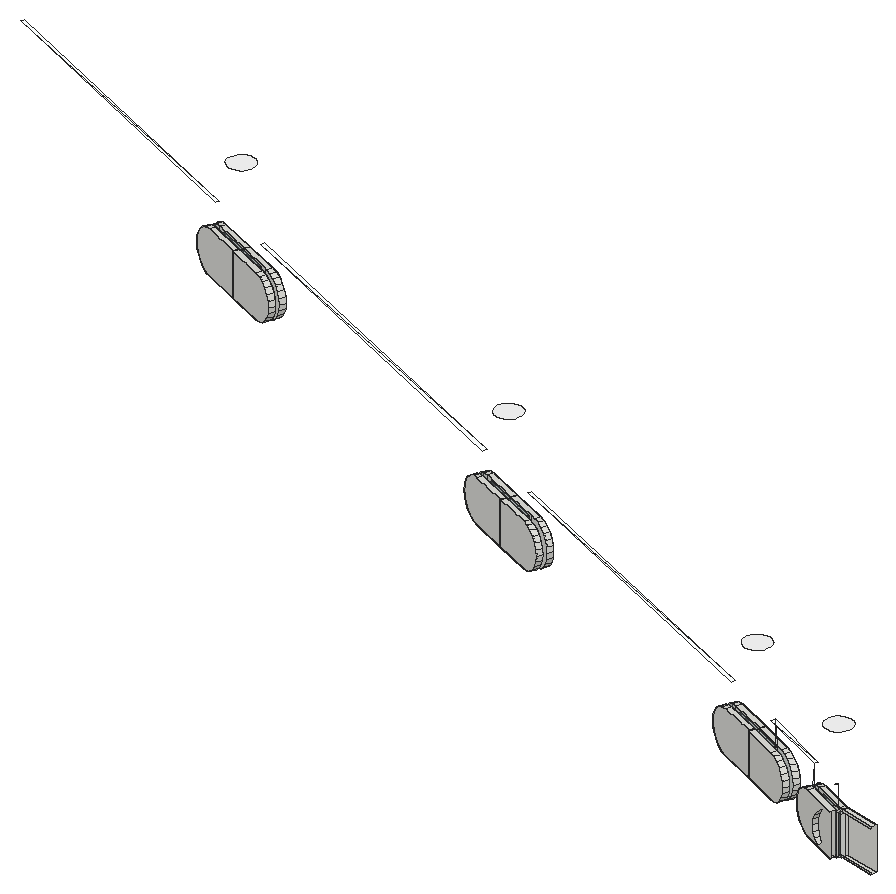
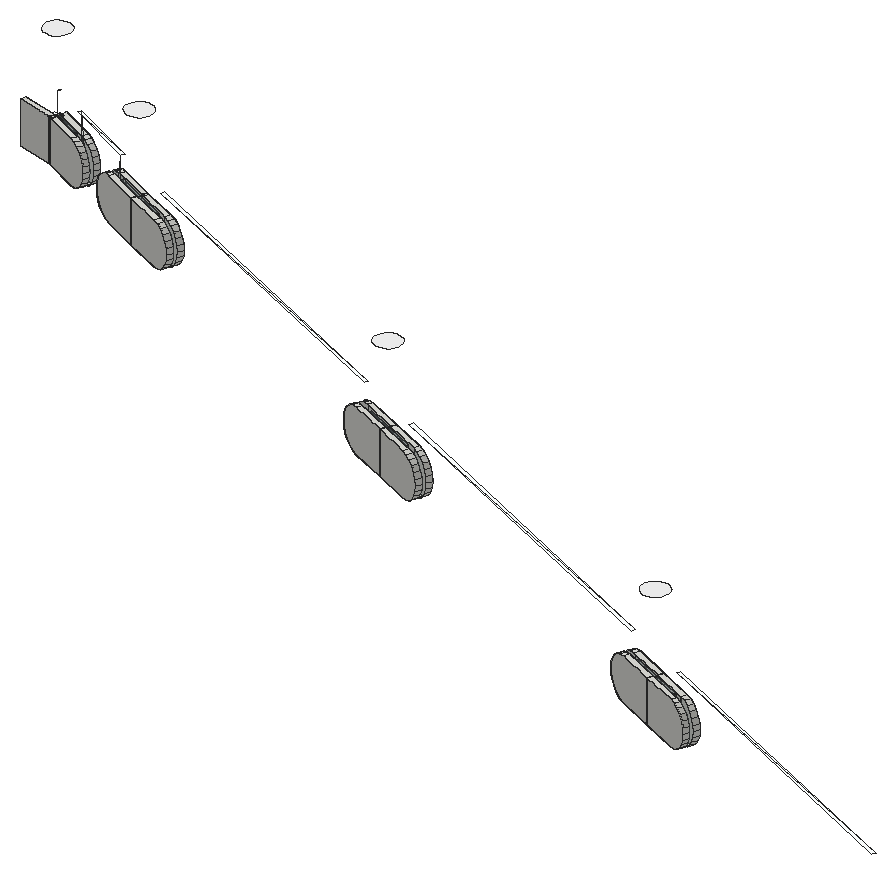
# SketchUp Ruby script. Lengths in inches.
U = 1.inch
M = Sketchup.active_model
def pt(a) = Geom::Point3d.new(a.map { |v| v * U })
def face(e, loops, mat)
  f = e.add_face(loops[0].map { |a| pt(a) })
  loops[1..].each { |l| e.add_face(l.map { |a| pt(a) }).erase! }
  f.material = f.back_material = mat if mat
  f
end
# faces: each face lists its corners as indices into pts; further lists are holes
def faces(e, pts, list, mat = nil) = list.each { |f| face(e, (f[0].is_a?(Array) ? f : [f]).map { |l| l.map { |i| pts[i] } }, mat) }
# xy, xz, yz: faces in a plane at the given z, y or x. An outline is a flat list of corners, or four numbers for a rectangle; further outlines are holes
def ring(l) = l.size == 4 ? [[l[0], l[1]], [l[2], l[1]], [l[2], l[3]], [l[0], l[3]]] : l.each_slice(2).to_a
def flat(e, list, mat, &to3) = list.each { |f| face(e, (f[0].is_a?(Array) ? f : [f]).map { |l| ring(l).map { |u, v| to3.(u, v) } }, mat) }
def xy(e, z, list, mat = nil) = flat(e, list, mat) { |x, y| [x, y, z] }
def xz(e, y, list, mat = nil) = flat(e, list, mat) { |x, z| [x, y, z] }
def yz(e, x, list, mat = nil) = flat(e, list, mat) { |y, z| [x, y, z] }
def lines(e, pts, list) = list.each { |a, b| e.add_line(pt(pts[a]), pt(pts[b])) }
# prism: a flat outline (further loops are holes) pulled along v
def prism(e, loops, v, mat = nil)
  f = face(e, loops, mat); d = Geom::Vector3d.new(v.map { |x| x * U })
  f.pushpull(f.normal.samedirection?(d) ? d.length : -d.length)
end
def box(e, o, s, mat = nil) = prism(e, [[o, [o[0] + s[0], o[1], o[2]], [o[0] + s[0], o[1] + s[1], o[2]], [o[0], o[1] + s[1], o[2]]]], [0, 0, s[2]], mat)
def at(x, y, z, deg = 0) = Geom::Transformation.translation(pt([x, y, z])) * Geom::Transformation.rotation(ORIGIN, Z_AXIS, deg.degrees)
def axes(o, x, y, z) = Geom::Transformation.new([*x, 0, *y, 0, *z, 0, *pt(o).to_a, 1])
def part(name) = M.definitions.add(name)
# library, detail: a bought-in or finely detailed component or shape, given as its bounding box
def library(name, o, s) = part(name).tap { |d| box(d.entities, o, s) }
def detail(e, o, s) = box(e.add_group.entities, o, s)
def put(e, d, t, mat = nil) = e.add_instance(d, t).tap { |i| i.material = mat if mat }
def group(e, t, mat = nil) = e.add_group.tap { |g| g.transformation = t; g.material = mat if mat }.entities
root = M.entities
M.materials.add("Glass_Safety_01").color = [204, 235, 244]
M.materials["Glass_Safety_01"].alpha = 0.1
M.materials.add("[Color_000]").color = [255, 255, 255]
xy(root,351.283,[[1021.879,1012.714,1020.123,1013.542,1020.24,1013.791,1022.021,1012.952,1022.02,1012.949,1021.935,1012.968],[1023.9,1012.74,1022.106,1013.132,1022.222,1013.379,1022.184,1013.397,1023.959,1013.009],[1022.105,1013.13,1022.095,1013.134,1022.106,1013.132],[1022.106,1013.132,1022.095,1013.134,1021.983,1013.1875,1022.035,1013.429,1022.184,1013.397,1022.222,1013.379],[1022.095,1013.134,1022.084,1013.137,1021.977,1013.16,1021.983,1013.1875],
  [1021.983,1013.1875,1020.324,1013.969,1020.442,1014.219,1022.184,1013.397,1022.035,1013.429],[1017.116,1014.96,1015.346,1015.795,1015.456,1016.048,1016.751,1015.437,1017.234,1015.209],[1017.318,1015.387,1016.835,1015.615,1015.537,1016.227,1015.655,1016.476,1017.435,1015.637],[1015.346,1015.795,1015.341,1015.797,1015.336,1015.8,1015.453,1016.049,1015.456,1016.048],[1015.336,1015.8,1013.541,1016.581,1013.651,1016.834,1015.453,1016.049],
  [1015.535,1016.228,1013.73,1017.014,1013.84,1017.267,1015.645,1016.481],[998.018,1023.342,996.213,1024.128,996.324,1024.38,997.958,1023.669,998.128,1023.594],[998.207,1023.775,998.037,1023.849,996.402,1024.561,996.512,1024.814,998.317,1024.028],[996.213,1024.128,994.409,1024.914,994.519,1025.167,996.324,1024.38],[996.402,1024.561,994.597,1025.347,994.707,1025.6,996.512,1024.814],
  [977.436,1032.306,975.631,1033.092,975.741,1033.345,977.388,1032.628,977.546,1032.559],[977.625,1032.739,977.466,1032.808,975.82,1033.525,975.93,1033.778,977.735,1032.992],[975.631,1033.092,973.826,1033.878,973.936,1034.131,975.741,1033.345],[975.82,1033.525,974.015,1034.311,974.125,1034.564,975.93,1033.778]])
xy(root,351.362,[[1022.319,1012.884,1022.042,1012.945,1022.063,1013.041,1022.105,1013.13,1022.095,1013.134,1022.361,1013.076],[1022.021,1012.952,1020.597,1013.623,1020.681,1013.801,1022.095,1013.134,1022.084,1013.137,1022.063,1013.041],[1022.063,1013.041,1022.084,1013.137,1022.095,1013.134,1022.105,1013.13],[1016.878,1015.377,1016.751,1015.437,1015.456,1016.048,1015.495,1016.138,1015.537,1016.227,1016.835,1015.615,1016.962,1015.555],[1015.455,1016.048,1015.453,1016.049,1015.495,1016.138,1015.456,1016.048],
  [1015.453,1016.049,1014.012,1016.677,1014.091,1016.857,1015.535,1016.228,1015.495,1016.138],[997.767,1023.752,996.324,1024.38,996.402,1024.561,997.846,1023.932],[996.324,1024.38,994.88,1025.009,994.958,1025.19,996.402,1024.561],[977.185,1032.716,975.741,1033.345,975.82,1033.525,977.264,1032.896],[975.741,1033.345,974.297,1033.974,974.376,1034.154,975.82,1033.525]],"Glass_Safety_01")
xy(root,353.33,[[1022.319,1012.884,1022.361,1013.076,1022.095,1013.134,1022.105,1013.13,1022.063,1013.041,1022.042,1012.945],[1022.021,1012.952,1022.063,1013.041,1022.084,1013.137,1022.095,1013.134,1020.681,1013.801,1020.597,1013.623],[1022.063,1013.041,1022.105,1013.13,1022.095,1013.134,1022.084,1013.137],[1016.878,1015.377,1016.962,1015.555,1016.835,1015.615,1015.537,1016.227,1015.495,1016.138,1015.456,1016.048,1016.751,1015.437],[1015.455,1016.048,1015.456,1016.048,1015.495,1016.138,1015.453,1016.049],
  [1015.453,1016.049,1015.495,1016.138,1015.535,1016.228,1014.091,1016.857,1014.012,1016.677],[997.767,1023.752,997.846,1023.932,996.402,1024.561,996.324,1024.38],[996.324,1024.38,996.402,1024.561,994.958,1025.19,994.88,1025.009],[977.185,1032.716,977.264,1032.896,975.82,1033.525,975.741,1033.345],[975.741,1033.345,975.82,1033.525,974.376,1034.154,974.297,1033.974]],"Glass_Safety_01")
xy(root,353.409,[[1021.879,1012.714,1021.935,1012.968,1022.02,1012.949,1022.021,1012.952,1020.24,1013.791,1020.123,1013.542],[1023.9,1012.74,1023.959,1013.009,1022.184,1013.397,1022.222,1013.379,1022.106,1013.132],[1022.105,1013.13,1022.106,1013.132,1022.095,1013.134],[1022.106,1013.132,1022.222,1013.379,1022.184,1013.397,1022.035,1013.429,1021.983,1013.1875,1022.095,1013.134],[1022.095,1013.134,1021.983,1013.1875,1021.977,1013.16,1022.084,1013.137],
  [1021.983,1013.1875,1022.035,1013.429,1022.184,1013.397,1020.442,1014.219,1020.324,1013.969],[1017.116,1014.96,1017.234,1015.209,1016.751,1015.437,1015.456,1016.048,1015.346,1015.795],[1017.318,1015.387,1017.435,1015.637,1015.655,1016.476,1015.537,1016.227,1016.835,1015.615,1017.005,1015.535],[1015.346,1015.795,1015.456,1016.048,1015.453,1016.049,1015.336,1015.8,1015.341,1015.797],[1015.336,1015.8,1015.453,1016.049,1013.651,1016.834,1013.541,1016.581],
  [1015.535,1016.228,1015.645,1016.481,1013.84,1017.267,1013.73,1017.014],[998.018,1023.342,998.128,1023.594,997.958,1023.669,996.324,1024.38,996.213,1024.128],[998.207,1023.775,998.317,1024.028,996.512,1024.814,996.402,1024.561,998.037,1023.849],[996.213,1024.128,996.324,1024.38,994.519,1025.167,994.409,1024.914],[996.402,1024.561,996.512,1024.814,994.707,1025.6,994.597,1025.347],
  [977.436,1032.306,977.546,1032.559,977.388,1032.628,975.741,1033.345,975.631,1033.092],[977.625,1032.739,977.735,1032.992,975.93,1033.778,975.82,1033.525,977.466,1032.808],[975.631,1033.092,975.741,1033.345,973.936,1034.131,973.826,1033.878],[975.82,1033.525,975.93,1033.778,974.125,1034.564,974.015,1034.311]])
xy(root,354.511,[[1021.935,1012.968,1021.977,1013.16,1021.928,1012.969],[1021.928,1012.969,1021.977,1013.16,1021.97,1013.162],[1020.24,1013.791,1020.324,1013.969,1016.751,1015.437],[1020.324,1013.969,1016.835,1015.615,1016.751,1015.437],[1013.651,1016.834,1013.73,1017.014,997.958,1023.669],
  [1013.73,1017.014,998.037,1023.849,997.958,1023.669],[994.519,1025.167,994.597,1025.347,977.388,1032.628],[994.597,1025.347,977.466,1032.808,977.388,1032.628],[973.936,1034.131,974.015,1034.311,958.914,1040.674],[974.015,1034.311,958.992,1040.854,958.914,1040.674]],"Glass_Safety_01")
xy(root,357.267,[[1022.108,1012.412,1022.269,1012.445,1022.416,1012.519,1022.539,1012.628,1022.63,1012.766,1022.681,1012.922,1022.691,1013.086,1022.658,1013.247,1022.584,1013.394,1022.475,1013.517,1022.338,1013.607,1022.182,1013.659,1022.018,1013.669,1021.857,1013.636,1021.71,1013.562,1021.587,1013.453,1021.496,1013.316,1021.444,1013.16,1021.435,1012.996,1021.468,1012.835,1021.541,1012.6875,1021.65,1012.565,1021.788,1012.474,1021.944,1012.422],[1015.54,1015.51,1015.701,1015.543,1015.848,1015.616,1015.971,1015.726,1016.062,1015.863,1016.114,1016.019,1016.124,1016.183,1016.09,1016.344,1016.017,1016.491,1015.908,1016.614,1015.77,1016.705,1015.614,1016.757,1015.45,1016.766,1015.289,1016.733,1015.142,1016.66,1015.019,1016.55,1014.929,1016.413,1014.877,1016.257,1014.867,1016.093,1014.9,1015.932,1014.974,1015.785,1015.083,1015.662,1015.22,1015.571,1015.376,1015.519],[996.408,1023.842,996.569,1023.875,996.716,1023.949,996.839,1024.058,996.929,1024.196,996.981,1024.352,996.991,1024.516,996.958,1024.677,996.884,1024.824,996.775,1024.947,996.638,1025.037,996.482,1025.089,996.318,1025.099,996.157,1025.066,996.01,1024.992,995.887,1024.883,995.796,1024.746,995.744,1024.59,995.735,1024.426,995.768,1024.265,995.841,1024.118,995.95,1023.995,996.088,1023.904,996.244,1023.852],[975.826,1032.807,975.987,1032.84,976.134,1032.913,976.257,1033.023,976.347,1033.16,976.399,1033.316,976.409,1033.48,976.376,1033.641,976.302,1033.788,976.193,1033.911,976.056,1034.002,975.9,1034.054,975.735,1034.063,975.574,1034.03,975.427,1033.957,975.304,1033.847,975.214,1033.71,975.162,1033.554,975.152,1033.39,975.185,1033.229,975.259,1033.082,975.368,1032.959,975.505,1032.868,975.661,1032.816]],"[Color_000]")
p = [[1021.903,1012.702,353.409],[1021.879,1012.714,353.409],[1020.123,1013.542,353.409],[1019.874,1013.659,353.373],[1019.642,1013.769,353.267],[1019.443,1013.863,353.098],
  [1019.29,1013.935,352.877],[1019.194,1013.98,352.621],[1019.161,1013.995,352.346],[1019.194,1013.98,352.071],[1019.29,1013.935,351.814],[1019.443,1013.863,351.594],
  [1019.642,1013.769,351.425],[1019.874,1013.659,351.319],[1020.123,1013.542,351.283],[1021.879,1012.714,351.283],[1021.903,1012.702,351.283],[1022.095,1013.134,351.362],
  [1022.361,1013.076,351.362],[1023.622,1012.801,351.362],[1023.9,1012.74,351.362],[1023.9,1012.74,351.283],[1022.106,1013.132,351.283],[1022.095,1013.134,351.283],
  [1022.084,1013.137,351.283],[1022.084,1013.137,351.362],[1022.063,1013.041,351.362],[1022.042,1012.945,351.362],[1022.042,1012.945,351.283],[1022.021,1012.952,351.283],
  [1020.24,1013.791,351.283],[1020.24,1013.791,353.409],[1022.021,1012.952,353.409],[1022.021,1012.952,353.33],[1020.597,1013.623,353.33],[1020.597,1013.623,351.362],
  [1022.021,1012.952,351.362],[1021.666,1013.027,353.373],[1021.928,1012.969,353.408],[1021.928,1012.969,351.284],[1021.666,1013.027,351.319],[1021.415,1013.081,351.425],
  [1021.2,1013.128,351.594],[1021.035,1013.164,351.814],[1020.932,1013.187,352.071],[1020.896,1013.195,352.346],[1020.932,1013.187,352.621],[1021.035,1013.164,352.877],
  [1021.2,1013.128,353.098],[1021.415,1013.081,353.267],[1022.184,1013.397,353.409],[1023.959,1013.009,353.409],[1023.959,1013.009,351.283],[1022.184,1013.397,351.283],
  [1022.035,1013.429,351.283],[1021.767,1013.488,351.319],[1021.516,1013.543,351.425],[1021.301,1013.59,351.594],[1021.136,1013.626,351.814],[1021.032,1013.649,352.071],
  [1020.997,1013.656,352.346],[1021.032,1013.649,352.621],[1021.136,1013.626,352.877],[1021.301,1013.59,353.098],[1021.516,1013.543,353.267],[1021.767,1013.488,353.373],
  [1022.035,1013.429,353.409],[1021.983,1013.1875,353.409],[1020.324,1013.969,353.409],[1020.324,1013.969,351.283],[1021.983,1013.1875,351.283],[1022.105,1013.13,351.283],
  [1022.105,1013.13,351.362],[1020.681,1013.801,351.362],[1020.681,1013.801,353.33],[1022.095,1013.134,353.33],[1022.105,1013.13,353.33],[1022.105,1013.13,353.409],
  [1022.095,1013.134,353.409],[1022.084,1013.137,353.409],[1021.977,1013.16,353.409],[1021.977,1013.16,351.283],[1022.084,1013.137,353.33],[1022.222,1013.379,351.283],
  [1022.222,1013.379,353.409],[1022.106,1013.132,353.409],[1021.708,1013.219,351.319],[1021.971,1013.161,351.284],[1021.971,1013.162,353.408],[1021.708,1013.219,353.373],
  [1021.457,1013.274,353.267],[1021.242,1013.321,353.098],[1021.077,1013.357,352.877],[1020.974,1013.379,352.621],[1020.938,1013.387,352.346],[1020.974,1013.379,352.071],
  [1021.077,1013.357,351.814],[1021.242,1013.321,351.594],[1021.457,1013.274,351.425],[1020.442,1014.219,351.283],[1020.193,1014.336,351.319],[1019.961,1014.445,351.425],
  [1019.762,1014.539,351.594],[1019.609,1014.611,351.814],[1019.513,1014.657,352.071],[1019.481,1014.672,352.346],[1019.513,1014.657,352.621],[1019.609,1014.611,352.877],
  [1019.762,1014.539,353.098],[1019.961,1014.445,353.267],[1020.193,1014.336,353.373],[1020.442,1014.219,353.409],[1019.992,1013.909,351.319],[1019.76,1014.018,351.425],
  [1019.764,1014.016,351.423],[1020.066,1013.873,353.384],[1020.076,1014.087,351.319],[1019.844,1014.196,351.425],[1019.645,1014.29,351.594],[1019.492,1014.362,351.814],
  [1019.396,1014.407,352.071],[1019.363,1014.423,352.346],[1019.396,1014.407,352.621],[1019.492,1014.362,352.877],[1019.645,1014.29,353.098],[1019.844,1014.196,353.267],
  [1020.076,1014.087,353.373],[1017.116,1014.96,353.409],[1015.346,1015.795,353.409],[1015.346,1015.795,351.283],[1017.116,1014.96,351.283],[1017.365,1014.843,351.319],
  [1017.597,1014.733,351.425],[1017.796,1014.639,351.594],[1017.949,1014.567,351.814],[1018.045,1014.522,352.071],[1018.078,1014.507,352.346],[1018.045,1014.522,352.621],
  [1017.949,1014.567,352.877],[1017.796,1014.639,353.098],[1017.597,1014.733,353.267],[1017.365,1014.843,353.373],[1017.483,1015.092,351.319],[1017.714,1014.983,351.425],
  [1016.751,1015.437,351.362],[1016.751,1015.437,351.283],[1017.234,1015.209,351.283],[1017.914,1014.889,351.594],[1018.066,1014.817,351.814],[1018.162,1014.771,352.071],
  [1018.195,1014.756,352.346],[1018.162,1014.771,352.621],[1018.066,1014.817,352.877],[1017.914,1014.889,353.098],[1017.714,1014.983,353.267],[1017.483,1015.092,353.373],
  [1017.234,1015.209,353.409],[1016.751,1015.437,353.409],[1016.751,1015.437,353.33],[1016.878,1015.377,353.33],[1016.878,1015.377,351.362],[1017.005,1015.535,353.409],
  [1017.333,1015.38,351.285],[1017.567,1015.27,351.319],[1017.798,1015.161,351.425],[1017.998,1015.067,351.594],[1018.15,1014.995,351.814],[1018.246,1014.949,352.071],
  [1018.279,1014.934,352.346],[1018.246,1014.949,352.621],[1018.15,1014.995,352.877],[1017.998,1015.067,353.098],[1017.798,1015.161,353.267],[1017.567,1015.27,353.373],
  [1017.318,1015.387,353.409],[1015.655,1016.476,353.409],[1017.435,1015.637,353.409],[1017.684,1015.519,353.373],[1017.916,1015.41,353.267],[1018.115,1015.316,353.098],
  [1018.268,1015.244,352.877],[1018.364,1015.199,352.621],[1018.397,1015.183,352.346],[1018.364,1015.199,352.071],[1018.268,1015.244,351.814],[1018.115,1015.316,351.594],
  [1017.916,1015.41,351.425],[1017.684,1015.519,351.319],[1017.435,1015.637,351.283],[1015.655,1016.476,351.283],[1017.318,1015.387,351.283],[1015.456,1016.048,351.283],
  [1015.456,1016.048,351.362],[1016.835,1015.615,353.409],[1016.835,1015.615,353.33],[1016.962,1015.555,353.33],[1016.962,1015.555,351.362],[1016.835,1015.615,351.362],
  [1016.835,1015.615,351.283],[1015.537,1016.227,351.283],[1015.537,1016.227,351.362],[1015.341,1015.797,353.409],[1015.336,1015.8,353.409],[1013.541,1016.581,353.409],
  [1013.289,1016.691,353.373],[1013.054,1016.793,353.267],[1012.852,1016.881,353.098],[1012.697,1016.949,352.877],[1012.6,1016.991,352.621],[1012.567,1017.006,352.346],
  [1012.6,1016.991,352.071],[1012.697,1016.949,351.814],[1012.852,1016.881,351.594],[1013.054,1016.793,351.425],[1013.289,1016.691,351.319],[1013.541,1016.581,351.283],
  [1015.336,1015.8,351.283],[1015.341,1015.797,351.283],[1015.456,1016.048,353.33],[1015.456,1016.048,353.409],[1015.453,1016.049,351.362],[1015.453,1016.049,351.283],
  [1015.453,1016.049,353.409],[1015.453,1016.049,353.33],[1013.651,1016.834,353.409],[1014.012,1016.677,353.33],[1014.012,1016.677,351.362],[1013.651,1016.834,351.283],
  [1013.399,1016.944,351.319],[1013.164,1017.046,351.425],[1012.962,1017.134,351.594],[1012.807,1017.201,351.814],[1012.71,1017.244,352.071],[1012.677,1017.258,352.346],
  [1012.71,1017.244,352.621],[1012.807,1017.201,352.877],[1012.962,1017.134,353.098],[1013.164,1017.046,353.267],[1013.399,1016.944,353.373],[1015.455,1016.048,351.362],
  [1015.535,1016.228,353.409],[1013.73,1017.014,353.409],[1013.73,1017.014,351.283],[1015.535,1016.228,351.283],[1015.535,1016.228,351.362],[1014.091,1016.857,351.362],
  [1014.091,1016.857,353.33],[1015.535,1016.228,353.33],[1015.537,1016.227,353.33],[1015.537,1016.227,353.409],[1015.645,1016.481,351.283],[1015.645,1016.481,353.409],
  [1013.84,1017.267,353.409],[1013.84,1017.267,351.283],[1013.588,1017.377,351.319],[1013.353,1017.479,351.425],[1013.151,1017.567,351.594],[1012.996,1017.635,351.814],
  [1012.898,1017.677,352.071],[1012.865,1017.691,352.346],[1012.898,1017.677,352.621],[1012.996,1017.635,352.877],[1013.151,1017.567,353.098],[1013.353,1017.479,353.267],
  [1013.588,1017.377,353.373],[1013.478,1017.124,351.319],[1013.242,1017.226,351.425],[1013.041,1017.314,351.594],[1012.886,1017.382,351.814],[1012.788,1017.424,352.071],
  [1012.755,1017.439,352.346],[1012.788,1017.424,352.621],[1012.886,1017.382,352.877],[1013.041,1017.314,353.098],[1013.242,1017.226,353.267],[1013.478,1017.124,353.373],
  [998.018,1023.342,353.409],[996.213,1024.128,353.409],[996.213,1024.128,351.283],[998.018,1023.342,351.283],[998.27,1023.232,351.319],[998.506,1023.13,351.425],
  [998.707,1023.042,351.594],[998.862,1022.974,351.814],[998.96,1022.932,352.071],[998.993,1022.917,352.346],[998.96,1022.932,352.621],[998.862,1022.974,352.877],
  [998.707,1023.042,353.098],[998.506,1023.13,353.267],[998.27,1023.232,353.373],[998.381,1023.485,351.319],[998.616,1023.382,351.425],[998.128,1023.594,351.283],
  [997.958,1023.669,351.283],[997.958,1023.669,353.409],[998.128,1023.594,353.409],[998.381,1023.485,353.373],[998.616,1023.382,353.267],[998.817,1023.294,353.098],
  [998.972,1023.227,352.877],[999.07,1023.184,352.621],[999.103,1023.17,352.346],[999.07,1023.184,352.071],[998.972,1023.227,351.814],[998.817,1023.294,351.594],
  [998.207,1023.775,353.409],[998.037,1023.849,353.409],[998.037,1023.849,351.283],[998.207,1023.775,351.283],[998.459,1023.665,351.319],[998.694,1023.563,351.425],
  [998.896,1023.475,351.594],[999.051,1023.407,351.814],[999.148,1023.365,352.071],[999.181,1023.35,352.346],[999.148,1023.365,352.621],[999.051,1023.407,352.877],
  [998.896,1023.475,353.098],[998.694,1023.563,353.267],[998.459,1023.665,353.373],[996.512,1024.814,353.409],[998.317,1024.028,353.409],[998.569,1023.918,353.373],
  [998.804,1023.815,353.267],[999.006,1023.727,353.098],[999.161,1023.66,352.877],[999.258,1023.618,352.621],[999.291,1023.603,352.346],[999.258,1023.618,352.071],
  [999.161,1023.66,351.814],[999.006,1023.727,351.594],[998.804,1023.815,351.425],[998.569,1023.918,351.319],[998.317,1024.028,351.283],[996.512,1024.814,351.283],
  [996.324,1024.38,353.409],[996.324,1024.38,351.283],[996.324,1024.38,351.362],[997.767,1023.752,351.362],[997.767,1023.752,353.33],[996.324,1024.38,353.33],
  [996.402,1024.561,351.283],[996.402,1024.561,353.409],[996.402,1024.561,353.33],[997.846,1023.932,353.33],[997.846,1023.932,351.362],[996.402,1024.561,351.362],
  [994.409,1024.914,353.409],[994.156,1025.024,353.373],[993.921,1025.126,353.267],[993.72,1025.214,353.098],[993.565,1025.281,352.877],[993.467,1025.324,352.621],
  [993.434,1025.338,352.346],[993.467,1025.324,352.071],[993.565,1025.281,351.814],[993.72,1025.214,351.594],[993.921,1025.126,351.425],[994.156,1025.024,351.319],
  [994.409,1024.914,351.283],[994.519,1025.167,351.283],[994.519,1025.167,353.409],[994.88,1025.009,353.33],[994.88,1025.009,351.362],[994.597,1025.347,353.409],
  [994.597,1025.347,351.283],[994.958,1025.19,351.362],[994.958,1025.19,353.33],[994.707,1025.6,353.409],[994.707,1025.6,351.283],[994.455,1025.71,351.319],
  [994.22,1025.812,351.425],[994.018,1025.9,351.594],[993.863,1025.967,351.814],[993.766,1026.01,352.071],[993.733,1026.024,352.346],[993.766,1026.01,352.621],
  [993.863,1025.967,352.877],[994.018,1025.9,353.098],[994.22,1025.812,353.267],[994.455,1025.71,353.373],[994.267,1025.276,351.319],[994.031,1025.379,351.425],
  [994.267,1025.276,353.373],[994.031,1025.379,353.267],[993.83,1025.467,353.098],[993.675,1025.534,352.877],[993.577,1025.577,352.621],[993.544,1025.591,352.346],
  [993.577,1025.577,352.071],[993.675,1025.534,351.814],[993.83,1025.467,351.594],[994.345,1025.457,351.319],[994.11,1025.559,351.425],[993.908,1025.647,351.594],
  [993.753,1025.715,351.814],[993.656,1025.757,352.071],[993.623,1025.771,352.346],[993.656,1025.757,352.621],[993.753,1025.715,352.877],[993.908,1025.647,353.098],
  [994.11,1025.559,353.267],[994.345,1025.457,353.373],[977.436,1032.306,353.409],[975.631,1033.092,353.409],[975.631,1033.092,351.283],[977.436,1032.306,351.283],
  [977.688,1032.196,351.319],[977.923,1032.094,351.425],[978.125,1032.006,351.594],[978.28,1031.938,351.814],[978.377,1031.896,352.071],[978.41,1031.882,352.346],
  [978.377,1031.896,352.621],[978.28,1031.938,352.877],[978.125,1032.006,353.098],[977.923,1032.094,353.267],[977.688,1032.196,353.373],[977.546,1032.559,351.283],
  [977.388,1032.628,351.283],[977.388,1032.628,353.409],[977.546,1032.559,353.409],[977.798,1032.449,353.373],[978.033,1032.346,353.267],[978.235,1032.259,353.098],
  [978.39,1032.191,352.877],[978.487,1032.149,352.621],[978.521,1032.134,352.346],[978.487,1032.149,352.071],[978.39,1032.191,351.814],[978.235,1032.259,351.594],
  [978.033,1032.346,351.425],[977.798,1032.449,351.319],[977.625,1032.739,353.409],[977.466,1032.808,353.409],[977.466,1032.808,351.283],[977.625,1032.739,351.283],
  [977.877,1032.629,351.319],[978.112,1032.527,351.425],[978.314,1032.439,351.594],[978.469,1032.372,351.814],[978.566,1032.329,352.071],[978.599,1032.315,352.346],
  [978.566,1032.329,352.621],[978.469,1032.372,352.877],[978.314,1032.439,353.098],[978.112,1032.527,353.267],[977.877,1032.629,353.373],[977.987,1032.882,351.319],
  [978.222,1032.78,351.425],[975.741,1033.345,353.409],[975.741,1033.345,351.283],[975.741,1033.345,351.362],[977.185,1032.716,351.362],[977.185,1032.716,353.33],
  [975.741,1033.345,353.33],[975.93,1033.778,353.409],[977.735,1032.992,353.409],[977.987,1032.882,353.373],[978.222,1032.78,353.267],[978.424,1032.692,353.098],
  [978.579,1032.624,352.877],[978.676,1032.582,352.621],[978.709,1032.567,352.346],[978.676,1032.582,352.071],[978.579,1032.624,351.814],[978.424,1032.692,351.594],
  [977.735,1032.992,351.283],[975.93,1033.778,351.283],[975.82,1033.525,351.283],[975.82,1033.525,353.409],[975.82,1033.525,353.33],[977.264,1032.896,353.33],
  [977.264,1032.896,351.362],[975.82,1033.525,351.362],[973.826,1033.878,353.409],[973.574,1033.988,353.373],[973.339,1034.09,353.267],[973.137,1034.178,353.098],
  [972.982,1034.246,352.877],[972.885,1034.288,352.621],[972.852,1034.303,352.346],[972.885,1034.288,352.071],[972.982,1034.246,351.814],[973.137,1034.178,351.594],
  [973.339,1034.09,351.425],[973.574,1033.988,351.319],[973.826,1033.878,351.283],[973.936,1034.131,351.283],[973.936,1034.131,353.409],[974.297,1033.974,353.33],
  [974.297,1033.974,351.362],[974.015,1034.311,353.409],[974.015,1034.311,351.283],[974.376,1034.154,351.362],[974.376,1034.154,353.33],[974.125,1034.564,353.409],
  [974.125,1034.564,351.283],[973.873,1034.674,351.319],[973.638,1034.776,351.425],[973.436,1034.864,351.594],[973.281,1034.931,351.814],[973.184,1034.974,352.071],
  [973.15,1034.988,352.346],[973.184,1034.974,352.621],[973.281,1034.931,352.877],[973.436,1034.864,353.098],[973.638,1034.776,353.267],[973.873,1034.674,353.373],
  [973.684,1034.241,351.319],[973.449,1034.343,351.425],[973.684,1034.241,353.373],[973.449,1034.343,353.267],[973.247,1034.431,353.098],[973.092,1034.498,352.877],
  [972.995,1034.541,352.621],[972.962,1034.555,352.346],[972.995,1034.541,352.071],[973.092,1034.498,351.814],[973.247,1034.431,351.594],[973.763,1034.421,351.319],
  [973.528,1034.523,351.425],[973.326,1034.611,351.594],[973.171,1034.679,351.814],[973.074,1034.721,352.071],[973.04,1034.736,352.346],[973.074,1034.721,352.621],
  [973.171,1034.679,352.877],[973.326,1034.611,353.098],[973.528,1034.523,353.267],[973.763,1034.421,353.373],[1022.063,1013.041,353.33],[1022.042,1012.945,353.33],
  [1022.361,1013.076,353.33],[1019.561,1014.112,351.594],[1019.992,1013.909,353.373],[1019.76,1014.018,353.267],[1019.561,1014.112,353.098],[1019.408,1014.184,352.877],
  [1019.312,1014.229,352.621],[1019.279,1014.245,352.346],[1019.312,1014.229,352.071],[1019.408,1014.184,351.814],[1015.455,1016.048,353.33],[1015.495,1016.138,351.362],
  [1015.495,1016.138,353.33],[1021.141,1012.859,351.594],[1020.976,1012.895,351.814],[1020.873,1012.918,352.071],[1020.837,1012.926,352.346],[1020.873,1012.918,352.621],
  [1020.976,1012.895,352.877],[1021.141,1012.859,353.098],[1023.9,1012.74,353.33],[1023.622,1012.801,353.33],[1023.9,1012.74,353.409],[1022.042,1012.945,353.409],
  [1021.977,1013.16,354.511],[1021.97,1013.162,354.511],[1020.24,1013.791,354.511],[1016.835,1015.615,354.511]]
faces(root,p,[[0,1,2,3,4,5,6,7,8,9,10,11,12,13,14,15,16],[17,18,19,20,21,22,23,24,25],[25,26,27,28,24],[29,30,31,32,33,34,35,36],[37,38,39,40,41,42,43,44,45,46,47,48,49],[50,51,52,53,54,55,56,57,58,59,60,61,62,63,64,65,66],[67,68,69,70,23,71,72,17,73,74,75,76,77,78],[79,80,81,24,25,82],
  [72,71,22,83,84,85,77,76],[86,87,88,89,90,91,92,93,94,95,96,97,98],[86,98,56,55],[87,86,55,54,70,81],[50,84,83,53,99,100,101,102,103,104,105,106,107,108,109,110,111],[112,30,14,13],[113,114,112,13,12],[69,116,100,99],
  [116,117,101,100],[127,128,129,130,131,132,133,134,135,136,137,138,139,140,141],[142,143,132,131],[146,142,131,130],[175,176,177,178,179,180,181,182,183,184,185,186,187,188,189],[164,163,187,186],[163,162,190,188,187],[191,192,144,145],
  [199,198,197,200],[128,201,202,203,204,205,206,207,208,209,210,211,212,213,214,215,216,217,129],[217,129,128,201,202,216],[191,192,218,219,128,129],[220,221,216,202,222,223],[224,222,223,225,226,220,221,227,228,229,230,231,232,233,234,235,236,237,238],[191,221,220,239,192],[222,219,218,192,191,221,220,223],
  [240,241,242,243,244,245,246,247],[199,200,248,249,175,189],[244,243,250,251,240,247],[252,251,250,253,254,255,256,257,258,259,260,261,262,263,264],[228,227,215,214],[229,228,214,213],[242,265,254,253],[265,266,255,254],
  [276,277,278,279,280,281,282,283,284,285,286,287,288,289,290],[291,292,281,280],[293,294,295,296,297,298,299,300,301,302,303,304,305,292,291],[293,291,280,279],[306,307,308,309,310,311,312,313,314,315,316,317,318,319,320],[321,322,323,324,325,326,327,328,329,330,331,332,333,334,335],[311,310,333,332],[336,295,294,337,338,339,340,341],
  [310,309,334,333],[342,308,307,343,344,345,346,347],[277,348,349,350,351,352,353,354,355,356,357,358,359,360,278],[338,337,278,277,336,341],[337,361,362,336,341,363,364,338],[343,365,366,342,347,367,368,344],[342,347,344,343,321,335],[369,321,335,370,371,372,373,374,375,376,377,378,379,380,381],
  [382,361,360,359],[383,382,359,358],[366,393,371,370],[393,394,372,371],[404,405,406,407,408,409,410,411,412,413,414,415,416,417,418],[419,420,421,422,423,424,425,426,427,428,429,430,431,432,433],[433,432,409,408],[419,433,408,407],
  [434,435,436,437,438,439,440,441,442,443,444,445,446,447,448],[439,438,449,450],[451,421,420,452,453,454,455,456],[457,458,459,460,461,462,463,464,465,466,467,450,449,468,469],[438,437,468,449],[470,436,435,471,472,473,474,475],[405,476,477,478,479,480,481,482,483,484,485,486,487,488,406],[453,452,406,405,451,456],
  [452,489,490,451,456,491,492,453],[471,493,494,470,475,495,496,472],[470,475,472,471,457,469],[497,457,469,498,499,500,501,502,503,504,505,506,507,508,509],[510,489,488,487],[511,510,487,486],[494,521,499,498],[521,522,500,499],
  [26,532,533,27],[98,97,57,56],[535,113,12,11],[117,118,102,101],[143,147,133,132],[165,164,186,185],[158,159,160,144],[230,229,213,212],
  [266,267,256,255],[292,305,282,281],[312,311,332,331],[392,383,358,357],[394,395,373,372],[432,431,410,409],[440,439,450,467],[520,511,486,485],
  [522,523,501,500],[43,42,547,548],[97,96,58,57],[543,535,11,10],[118,119,103,102],[147,148,134,133],[166,165,185,184],[231,230,212,211],
  [267,268,257,256],[305,304,283,282],[313,312,331,330],[391,392,357,356],[395,396,374,373],[431,430,411,410],[441,440,467,466],[519,520,485,484],
  [523,524,502,501],[44,43,548,549],[96,95,59,58],[542,543,10,9],[119,120,104,103],[148,149,135,134],[167,166,184,183],[232,231,211,210],
  [268,269,258,257],[304,303,284,283],[314,313,330,329],[390,391,356,355],[396,397,375,374],[430,429,412,411],[442,441,466,465],[518,519,484,483],
  [524,525,503,502],[45,44,549,550],[95,94,60,59],[541,542,9,8],[120,121,105,104],[149,150,136,135],[168,167,183,182],[233,232,210,209],
  [269,270,259,258],[303,302,285,284],[315,314,329,328],[389,390,355,354],[397,398,376,375],[429,428,413,412],[443,442,465,464],[517,518,483,482],
  [525,526,504,503],[46,45,550,551],[94,93,61,60],[540,541,8,7],[121,122,106,105],[150,151,137,136],[169,168,182,181],[234,233,209,208],
  [270,271,260,259],[302,301,286,285],[316,315,328,327],[388,389,354,353],[398,399,377,376],[428,427,414,413],[444,443,464,463],[516,517,482,481],
  [526,527,505,504],[47,46,551,552],[93,92,62,61],[539,540,7,6],[122,123,107,106],[151,152,138,137],[170,169,181,180],[235,234,208,207],
  [271,272,261,260],[301,300,287,286],[317,316,327,326],[387,388,353,352],[399,400,378,377],[427,426,415,414],[445,444,463,462],[515,516,481,480],
  [527,528,506,505],[48,47,552,553],[92,91,63,62],[538,539,6,5],[123,124,108,107],[152,153,139,138],[171,170,180,179],[236,235,207,206],
  [272,273,262,261],[300,299,288,287],[318,317,326,325],[386,387,352,351],[400,401,379,378],[426,425,416,415],[446,445,462,461],[514,515,480,479],
  [528,529,507,506],[91,90,64,63],[537,538,5,4],[124,125,109,108],[153,154,140,139],[172,171,179,178],[237,236,206,205],[273,274,263,262],
  [299,298,289,288],[319,318,325,324],[385,386,351,350],[401,402,380,379],[425,424,417,416],[447,446,461,460],[513,514,479,478],[529,530,508,507],
  [554,555,534,75,82,79,78,85,556],[557,533,532,82,79],[90,89,65,64],[536,537,4,3],[125,126,110,109],[154,155,141,140],[173,172,178,177],[157,158,218,219],
  [248,194,193,249],[544,223,222,219,218],[238,237,205,204],[274,275,264,263],[298,297,290,289],[320,319,324,323],[384,385,350,349],[402,403,381,380],
  [424,423,418,417],[448,447,460,459],[512,513,478,477],[530,531,509,508],[88,80,67,66,65,89],[31,115,536,3,2],[126,68,111,110],[155,156,127,141],
  [174,173,177,176],[224,238,204,203],[275,241,252,264],[297,296,276,290],[306,320,323,322],[362,384,349,348],[403,365,369,381],[423,422,404,418],
  [434,448,459,458],[490,512,477,476],[531,493,497,509]])
faces(root,p,[[80,81,87,88],[31,30,112,114,115],[68,69,116,117,118,119,120,121,122,123,124,125,126],[144,145,146,142,143,147,148,149,150,151,152,153,154,155,156,157,158,159,160],[161,162,163,164,165,166,167,168,169,170,171,172,173,174],[162,161,193,194,195,196,197,198,190],[227,224,238,237,236,235,234,233,232,231,230,229,228],[241,242,265,266,267,268,269,270,271,272,273,274,275],
  [361,362,384,385,386,387,388,389,390,391,392,383,382],[365,366,393,394,395,396,397,398,399,400,401,402,403],[489,490,512,513,514,515,516,517,518,519,520,511,510],[493,494,521,522,523,524,525,526,527,528,529,530,531],[34,33,36,35],[26,532,33,36],[532,26,72,76],[26,25,82,532],
  [76,75,74,73,17,72],[82,75,534,18,17,25],[34,74,73,35],[114,115,536,537,538,539,540,541,542,543,535,113],[144,192,218,158],[158,144,160,159],[159,160,196,195],[194,248,200,197],
  [197,194,195,196],[225,223,220,226],[239,220,223,544,218,192],[545,546,218,192],[223,546,545,220],[200,545,546,248],[546,545,244,247],[247,246,245,244],
  [245,226,225,246],[341,340,339,338],[340,339,346,345],[345,344,347,346],[363,341,338,364],[341,344,347,338],[344,368,367,347],[368,367,364,363],
  [456,455,454,453],[455,454,474,473],[473,472,475,474],[491,456,453,492],[456,472,475,453],[472,496,495,475],[496,495,492,491],[558,80,88,559],
  [560,115,31],[561,161,193]],"Glass_Safety_01")
